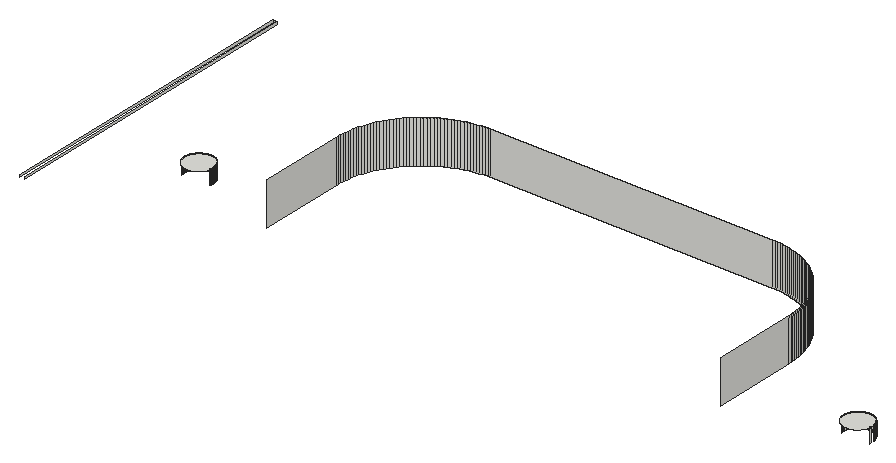
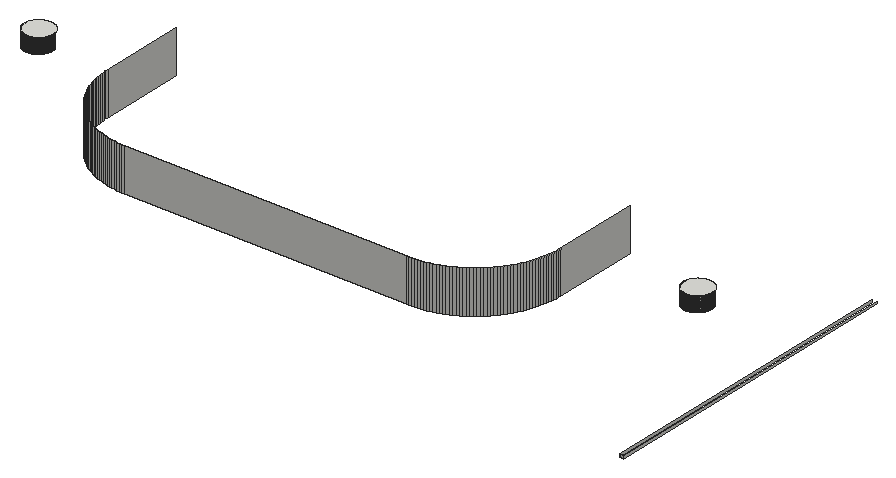
# SketchUp Ruby script. Lengths in inches.
U = 1.inch
M = Sketchup.active_model
def pt(a) = Geom::Point3d.new(a.map { |v| v * U })
def face(e, loops, mat)
  f = e.add_face(loops[0].map { |a| pt(a) })
  loops[1..].each { |l| e.add_face(l.map { |a| pt(a) }).erase! }
  f.material = f.back_material = mat if mat
  f
end
# faces: each face lists its corners as indices into pts; further lists are holes
def faces(e, pts, list, mat = nil) = list.each { |f| face(e, (f[0].is_a?(Array) ? f : [f]).map { |l| l.map { |i| pts[i] } }, mat) }
# xy, xz, yz: faces in a plane at the given z, y or x. An outline is a flat list of corners, or four numbers for a rectangle; further outlines are holes
def ring(l) = l.size == 4 ? [[l[0], l[1]], [l[2], l[1]], [l[2], l[3]], [l[0], l[3]]] : l.each_slice(2).to_a
def flat(e, list, mat, &to3) = list.each { |f| face(e, (f[0].is_a?(Array) ? f : [f]).map { |l| ring(l).map { |u, v| to3.(u, v) } }, mat) }
def xy(e, z, list, mat = nil) = flat(e, list, mat) { |x, y| [x, y, z] }
def xz(e, y, list, mat = nil) = flat(e, list, mat) { |x, z| [x, y, z] }
def yz(e, x, list, mat = nil) = flat(e, list, mat) { |y, z| [x, y, z] }
def lines(e, pts, list) = list.each { |a, b| e.add_line(pt(pts[a]), pt(pts[b])) }
# prism: a flat outline (further loops are holes) pulled along v
def prism(e, loops, v, mat = nil)
  f = face(e, loops, mat); d = Geom::Vector3d.new(v.map { |x| x * U })
  f.pushpull(f.normal.samedirection?(d) ? d.length : -d.length)
end
def box(e, o, s, mat = nil) = prism(e, [[o, [o[0] + s[0], o[1], o[2]], [o[0] + s[0], o[1] + s[1], o[2]], [o[0], o[1] + s[1], o[2]]]], [0, 0, s[2]], mat)
def at(x, y, z, deg = 0) = Geom::Transformation.translation(pt([x, y, z])) * Geom::Transformation.rotation(ORIGIN, Z_AXIS, deg.degrees)
def axes(o, x, y, z) = Geom::Transformation.new([*x, 0, *y, 0, *z, 0, *pt(o).to_a, 1])
def part(name) = M.definitions.add(name)
# library, detail: a bought-in or finely detailed component or shape, given as its bounding box
def library(name, o, s) = part(name).tap { |d| box(d.entities, o, s) }
def detail(e, o, s) = box(e.add_group.entities, o, s)
def put(e, d, t, mat = nil) = e.add_instance(d, t).tap { |i| i.material = mat if mat }
def group(e, t, mat = nil) = e.add_group.tap { |g| g.transformation = t; g.material = mat if mat }.entities
root = M.entities
xy(root,351,[[44.84,249,44.76,249.01,44.6875,249.02,44.61,249.03,44.45,249.05,44.375,249.07,44.3,249.08,44.22,249.1,44.15,249.125,44.07,249.15,44,249.17,43.92,249.2,43.71,249.29,43.64,249.33,43.57,249.36,43.43,249.44,43.37,249.48,43.3,249.53,43.24,249.57,43.17,249.62,42.93,249.82,42.88,249.88,42.77,249.99,42.62,250.17,42.57,250.24,42.53,250.3,42.48,250.37,42.44,250.43,42.36,250.57,42.33,250.64,42.29,250.71,42.23,250.85,42.2,250.93,42.17,251,42.15,251.07,42.125,251.15,42.1,251.22,42.08,251.3,42.07,251.375,42.05,251.45,42.03,251.61,42.02,251.6875,42.01,251.76,42,251.84,42,252.16,42.01,252.24,42.02,252.3125,42.03,252.39,42.05,252.55,42.07,252.625,42.08,252.7,42.1,252.78,42.125,252.85,42.15,252.93,42.17,253,42.2,253.08,42.29,253.29,42.33,253.36,42.36,253.43,42.44,253.57,42.48,253.63,42.53,253.7,42.57,253.76,42.62,253.83,42.82,254.07,42.88,254.12,42.99,254.23,43.17,254.38,43.24,254.43,43.3,254.47,43.37,254.52,43.43,254.56,43.57,254.64,43.64,254.67,43.71,254.71,43.85,254.77,43.93,254.8,44,254.83,44.07,254.85,44.15,254.875,44.22,254.9,44.3,254.92,44.375,254.93,44.45,254.95,44.61,254.97,44.6875,254.98,44.76,254.99,44.84,255,45.16,255,45.24,254.99,45.3125,254.98,45.39,254.97,45.55,254.95,45.625,254.93,45.7,254.92,45.78,254.9,45.85,254.875,45.93,254.85,46,254.83,46.08,254.8,46.29,254.71,46.36,254.67,46.43,254.64,46.57,254.56,46.63,254.52,46.7,254.47,46.76,254.43,46.83,254.38,47.07,254.18,47.12,254.12,47.23,254.01,47.38,253.83,47.43,253.76,47.47,253.7,47.52,253.63,47.56,253.57,47.64,253.43,47.67,253.36,47.71,253.29,47.77,253.15,47.8,253.07,47.83,253,47.85,252.93,47.875,252.85,47.9,252.78,47.92,252.7,47.93,252.625,47.95,252.55,47.97,252.39,47.98,252.3125,47.99,252.24,48,252.16,48,251.84,47.99,251.76,47.98,251.6875,47.97,251.61,47.95,251.45,47.93,251.375,47.92,251.3,47.9,251.22,47.875,251.15,47.85,251.07,47.83,251,47.8,250.92,47.71,250.71,47.67,250.64,47.64,250.57,47.56,250.43,47.52,250.37,47.47,250.3,47.43,250.24,47.38,250.17,47.18,249.93,47.12,249.88,47.01,249.77,46.83,249.62,46.76,249.57,46.7,249.53,46.63,249.48,46.57,249.44,46.43,249.36,46.36,249.33,46.29,249.29,46.15,249.23,46.07,249.2,46,249.17,45.93,249.15,45.85,249.125,45.78,249.1,45.7,249.08,45.625,249.07,45.55,249.05,45.39,249.03,45.3125,249.02,45.24,249.01,45.16,249],[182.84,249,182.76,249.01,182.6875,249.02,182.61,249.03,182.45,249.05,182.375,249.07,182.3,249.08,182.22,249.1,182.15,249.125,182.07,249.15,182,249.17,181.92,249.2,181.71,249.29,181.64,249.33,181.57,249.36,181.43,249.44,181.37,249.48,181.3,249.53,181.24,249.57,181.17,249.62,180.93,249.82,180.88,249.88,180.77,249.99,180.62,250.17,180.57,250.24,180.53,250.3,180.48,250.37,180.44,250.43,180.36,250.57,180.33,250.64,180.29,250.71,180.23,250.85,180.2,250.93,180.17,251,180.15,251.07,180.125,251.15,180.1,251.22,180.08,251.3,180.07,251.375,180.05,251.45,180.03,251.61,180.02,251.6875,180.01,251.76,180,251.84,180,252.16,180.01,252.24,180.02,252.3125,180.03,252.39,180.05,252.55,180.07,252.625,180.08,252.7,180.1,252.78,180.125,252.85,180.15,252.93,180.17,253,180.2,253.08,180.29,253.29,180.33,253.36,180.36,253.43,180.44,253.57,180.48,253.63,180.53,253.7,180.57,253.76,180.62,253.83,180.82,254.07,180.88,254.12,180.99,254.23,181.17,254.38,181.24,254.43,181.3,254.47,181.37,254.52,181.43,254.56,181.57,254.64,181.64,254.67,181.71,254.71,181.85,254.77,181.93,254.8,182,254.83,182.07,254.85,182.15,254.875,182.22,254.9,182.3,254.92,182.375,254.93,182.45,254.95,182.61,254.97,182.6875,254.98,182.76,254.99,182.84,255,183.16,255,183.24,254.99,183.3125,254.98,183.39,254.97,183.55,254.95,183.625,254.93,183.7,254.92,183.78,254.9,183.85,254.875,183.93,254.85,184,254.83,184.08,254.8,184.29,254.71,184.36,254.67,184.43,254.64,184.57,254.56,184.63,254.52,184.7,254.47,184.76,254.43,184.83,254.38,185.07,254.18,185.12,254.12,185.23,254.01,185.38,253.83,185.43,253.76,185.47,253.7,185.52,253.63,185.56,253.57,185.64,253.43,185.67,253.36,185.71,253.29,185.77,253.15,185.8,253.07,185.83,253,185.85,252.93,185.875,252.85,185.9,252.78,185.92,252.7,185.93,252.625,185.95,252.55,185.97,252.39,185.98,252.3125,185.99,252.24,186,252.16,186,251.84,185.99,251.76,185.98,251.6875,185.97,251.61,185.95,251.45,185.93,251.375,185.92,251.3,185.9,251.22,185.875,251.15,185.85,251.07,185.83,251,185.8,250.92,185.71,250.71,185.67,250.64,185.64,250.57,185.56,250.43,185.52,250.37,185.47,250.3,185.43,250.24,185.38,250.17,185.18,249.93,185.12,249.88,185.01,249.77,184.83,249.62,184.76,249.57,184.7,249.53,184.63,249.48,184.57,249.44,184.43,249.36,184.36,249.33,184.29,249.29,184.15,249.23,184.07,249.2,184,249.17,183.93,249.15,183.85,249.125,183.78,249.1,183.7,249.08,183.625,249.07,183.55,249.05,183.39,249.03,183.3125,249.02,183.24,249.01,183.16,249]])
xz(root,255,[[44.84,348,44.92,351],[44.92,348,45,351],[45,348,45.08,351],[45.08,348,45.16,351],[182.84,348,182.92,351],
  [182.92,348,183,351],[183,348,183.08,351],[183.08,348,183.16,351]])
xz(root,282,[[82,348,141,357]])
xz(root,300,[[22,348,23,348.5]])
yz(root,22,[[234,348,300,348.5]])
yz(root,23,[[234,348,300,348.5]])
yz(root,42,[[251.84,348,251.92,351],[251.92,348,252,351],[252,348,252.08,351],[252.08,348,252.16,351]])
yz(root,48,[[251.84,348,251.92,351],[251.92,348,252,351],[252,348,252.08,351],[252.08,348,252.16,351]])
yz(root,64,[[246,348,264,357]])
yz(root,159,[[246,348,264,357]])
yz(root,180,[[251.84,348,251.92,351],[251.92,348,252,351],[252,348,252.08,351],[252.08,348,252.16,351]])
p = [[42.08,251.3,348],[42.07,251.375,348],[42.07,251.375,351],[42.08,251.3,351],[47.93,251.375,348],[47.92,251.3,348],
  [47.92,251.3,351],[47.93,251.375,351],[180.08,251.3,348],[180.07,251.375,348],[180.07,251.375,351],[180.08,251.3,351],
  [42.05,251.45,348],[42.05,251.45,351],[47.95,251.45,348],[47.95,251.45,351],[180.05,251.45,348],[180.05,251.45,351],
  [185.95,251.45,348],[185.93,251.375,348],[185.93,251.375,351],[185.95,251.45,351],[42.04,251.53,348],[42.03,251.61,348],
  [42.03,251.61,351],[42.04,251.53,351],[47.96,251.53,348],[47.96,251.53,351],[47.97,251.61,348],[47.97,251.61,351],
  [180.04,251.53,348],[180.03,251.61,348],[180.03,251.61,351],[180.04,251.53,351],[185.96,251.53,348],[185.96,251.53,351],
  [185.97,251.61,348],[185.97,251.61,351],[42.02,251.6875,348],[42.02,251.6875,351],[47.98,251.6875,348],[47.98,251.6875,351],
  [180.02,251.6875,348],[180.02,251.6875,351],[185.98,251.6875,348],[185.98,251.6875,351],[42.01,251.76,348],[42.01,251.76,351],
  [47.99,251.76,348],[47.99,251.76,351],[180.01,251.76,348],[180.01,251.76,351],[42,251.84,348],[42,251.84,351],
  [48,251.84,348],[48,251.84,351],[180,251.84,348],[180,251.84,351],[42,252.16,348],[42.01,252.24,348],
  [42.01,252.24,351],[42,252.16,351],[42.02,252.3125,348],[42.02,252.3125,351],[47.98,252.3125,348],[47.99,252.24,348],
  [47.99,252.24,351],[47.98,252.3125,351],[48,252.16,348],[48,252.16,351],[180,252.16,348],[180.01,252.24,348],
  [180.01,252.24,351],[180,252.16,351],[180.02,252.3125,348],[180.02,252.3125,351],[42.03,252.39,348],[42.03,252.39,351],
  [47.97,252.39,348],[47.97,252.39,351],[180.03,252.39,348],[180.03,252.39,351],[42.04,252.47,348],[42.04,252.47,351],
  [47.96,252.47,348],[47.96,252.47,351],[180.04,252.47,348],[180.04,252.47,351],[185.96,252.47,348],[185.97,252.39,348],
  [185.97,252.39,351],[185.96,252.47,351],[42.05,252.55,348],[42.05,252.55,351],[42.07,252.625,348],[42.07,252.625,351],
  [47.93,252.625,348],[47.95,252.55,348],[47.95,252.55,351],[47.93,252.625,351],[180.05,252.55,348],[180.05,252.55,351],
  [180.07,252.625,348],[180.07,252.625,351],[185.93,252.625,348],[185.95,252.55,348],[185.95,252.55,351],[185.93,252.625,351],
  [42.08,252.7,348],[42.08,252.7,351],[47.92,252.7,348],[47.92,252.7,351],[180.08,252.7,348],[180.08,252.7,351],
  [185.92,252.7,348],[185.92,252.7,351],[42.1,252.78,348],[42.1,252.78,351],[47.9,252.78,348],[47.9,252.78,351],
  [180.1,252.78,348],[180.1,252.78,351],[185.9,252.78,348],[185.9,252.78,351],[42.125,252.85,348],[42.125,252.85,351],
  [47.875,252.85,348],[47.875,252.85,351],[180.125,252.85,348],[180.125,252.85,351],[185.875,252.85,348],[185.875,252.85,351],
  [42.15,252.93,348],[42.15,252.93,351],[42.17,253,348],[42.17,253,351],[47.83,253,348],[47.85,252.93,348],
  [47.85,252.93,351],[47.83,253,351],[180.15,252.93,348],[180.15,252.93,351],[180.17,253,348],[180.17,253,351],
  [185.83,253,348],[185.85,252.93,348],[185.85,252.93,351],[185.83,253,351],[42.2,253.08,348],[42.2,253.08,351],
  [47.8,253.07,348],[47.8,253.07,351],[180.2,253.08,348],[180.2,253.08,351],[185.8,253.07,348],[185.8,253.07,351],
  [42.23,253.15,348],[42.23,253.15,351],[42.26,253.22,348],[42.26,253.22,351],[47.74,253.22,348],[47.77,253.15,348],
  [47.77,253.15,351],[47.74,253.22,351],[180.23,253.15,348],[180.23,253.15,351],[180.26,253.22,348],[180.26,253.22,351],
  [185.74,253.22,348],[185.77,253.15,348],[185.77,253.15,351],[185.74,253.22,351],[42.29,253.29,348],[42.29,253.29,351],
  [47.71,253.29,348],[47.71,253.29,351],[180.29,253.29,348],[180.29,253.29,351],[185.71,253.29,348],[185.71,253.29,351],
  [42.33,253.36,348],[42.33,253.36,351],[47.67,253.36,348],[47.67,253.36,351],[180.33,253.36,348],[180.33,253.36,351],
  [185.67,253.36,348],[185.67,253.36,351],[42.36,253.43,348],[42.36,253.43,351],[42.4,253.5,348],[42.4,253.5,351],
  [47.6,253.5,348],[47.64,253.43,348],[47.64,253.43,351],[47.6,253.5,351],[180.36,253.43,348],[180.36,253.43,351],
  [180.4,253.5,348],[180.4,253.5,351],[185.6,253.5,348],[185.64,253.43,348],[185.64,253.43,351],[185.6,253.5,351],
  [42.44,253.57,348],[42.44,253.57,351],[47.56,253.57,348],[47.56,253.57,351],[180.44,253.57,348],[180.44,253.57,351],
  [185.56,253.57,348],[185.56,253.57,351],[42.48,253.63,348],[42.48,253.63,351],[42.53,253.7,348],[42.53,253.7,351],
  [47.47,253.7,348],[47.52,253.63,348],[47.52,253.63,351],[47.47,253.7,351],[180.48,253.63,348],[180.48,253.63,351],
  [180.53,253.7,348],[180.53,253.7,351],[185.47,253.7,348],[185.52,253.63,348],[185.52,253.63,351],[185.47,253.7,351],
  [42.57,253.76,348],[42.57,253.76,351],[47.43,253.76,348],[47.43,253.76,351],[180.57,253.76,348],[180.57,253.76,351],
  [185.43,253.76,348],[185.43,253.76,351],[42.62,253.83,348],[42.62,253.83,351],[42.67,253.89,348],[42.67,253.89,351],
  [47.33,253.89,348],[47.38,253.83,348],[47.38,253.83,351],[47.33,253.89,351],[180.62,253.83,348],[180.62,253.83,351],
  [180.67,253.89,348],[180.67,253.89,351],[185.33,253.89,348],[185.38,253.83,348],[185.38,253.83,351],[185.33,253.89,351],
  [42.72,253.95,348],[42.72,253.95,351],[42.77,254.01,348],[42.77,254.01,351],[47.23,254.01,348],[47.28,253.95,348],
  [47.28,253.95,351],[47.23,254.01,351],[180.72,253.95,348],[180.72,253.95,351],[180.77,254.01,348],[180.77,254.01,351],
  [185.23,254.01,348],[185.28,253.95,348],[185.28,253.95,351],[185.23,254.01,351],[42.82,254.07,348],[42.82,254.07,351],
  [47.18,254.06,348],[47.18,254.06,351],[180.82,254.07,348],[180.82,254.07,351],[185.18,254.06,348],[185.18,254.06,351],
  [42.88,254.12,348],[42.88,254.12,351],[42.94,254.18,348],[42.94,254.18,351],[47.07,254.18,348],[47.12,254.12,348],
  [47.12,254.12,351],[47.07,254.18,351],[180.88,254.12,348],[180.88,254.12,351],[180.94,254.18,348],[180.94,254.18,351],
  [185.07,254.18,348],[185.12,254.12,348],[185.12,254.12,351],[185.07,254.18,351],[42.99,254.23,348],[42.99,254.23,351],
  [43.05,254.28,348],[43.05,254.28,351],[46.95,254.28,348],[47.01,254.23,348],[47.01,254.23,351],[46.95,254.28,351],
  [180.99,254.23,348],[180.99,254.23,351],[181.05,254.28,348],[181.05,254.28,351],[184.95,254.28,348],[185.01,254.23,348],
  [185.01,254.23,351],[184.95,254.28,351],[43.11,254.33,348],[43.11,254.33,351],[43.17,254.38,348],[43.17,254.38,351],
  [46.83,254.38,348],[46.89,254.33,348],[46.89,254.33,351],[46.83,254.38,351],[181.11,254.33,348],[181.11,254.33,351],
  [181.17,254.38,348],[181.17,254.38,351],[184.83,254.38,348],[184.89,254.33,348],[184.89,254.33,351],[184.83,254.38,351],
  [43.24,254.43,348],[43.24,254.43,351],[43.3,254.47,348],[43.3,254.47,351],[46.7,254.47,348],[46.76,254.43,348],
  [46.76,254.43,351],[46.7,254.47,351],[181.24,254.43,348],[181.24,254.43,351],[181.3,254.47,348],[181.3,254.47,351],
  [184.7,254.47,348],[184.76,254.43,348],[184.76,254.43,351],[184.7,254.47,351],[43.37,254.52,348],[43.37,254.52,351],
  [43.43,254.56,348],[43.43,254.56,351],[46.57,254.56,348],[46.63,254.52,348],[46.63,254.52,351],[46.57,254.56,351],
  [181.37,254.52,348],[181.37,254.52,351],[181.43,254.56,348],[181.43,254.56,351],[184.57,254.56,348],[184.63,254.52,348],
  [184.63,254.52,351],[184.57,254.56,351],[43.5,254.6,348],[43.5,254.6,351],[43.57,254.64,348],[43.57,254.64,351],
  [43.64,254.67,348],[43.64,254.67,351],[46.36,254.67,348],[46.43,254.64,348],[46.43,254.64,351],[46.36,254.67,351],
  [46.5,254.6,348],[46.5,254.6,351],[181.5,254.6,348],[181.5,254.6,351],[181.57,254.64,348],[181.57,254.64,351],
  [181.64,254.67,348],[181.64,254.67,351],[184.36,254.67,348],[184.43,254.64,348],[184.43,254.64,351],[184.36,254.67,351],
  [184.5,254.6,348],[184.5,254.6,351],[43.71,254.71,348],[43.71,254.71,351],[43.78,254.74,348],[43.78,254.74,351],
  [43.85,254.77,348],[43.85,254.77,351],[46.15,254.77,348],[46.22,254.74,348],[46.22,254.74,351],[46.15,254.77,351],
  [46.29,254.71,348],[46.29,254.71,351],[181.71,254.71,348],[181.71,254.71,351],[181.78,254.74,348],[181.78,254.74,351],
  [181.85,254.77,348],[181.85,254.77,351],[184.15,254.77,348],[184.22,254.74,348],[184.22,254.74,351],[184.15,254.77,351],
  [184.29,254.71,348],[184.29,254.71,351],[43.93,254.8,348],[43.93,254.8,351],[44,254.83,348],[44,254.83,351],
  [44.07,254.85,348],[44.07,254.85,351],[45.93,254.85,348],[46,254.83,348],[46,254.83,351],[45.93,254.85,351],
  [46.08,254.8,348],[46.08,254.8,351],[181.93,254.8,348],[181.93,254.8,351],[182,254.83,348],[182,254.83,351],
  [182.07,254.85,348],[182.07,254.85,351],[183.93,254.85,348],[184,254.83,348],[184,254.83,351],[183.93,254.85,351],
  [184.08,254.8,348],[184.08,254.8,351],[44.15,254.875,348],[44.15,254.875,351],[44.22,254.9,348],[44.22,254.9,351],
  [44.3,254.92,348],[44.3,254.92,351],[44.375,254.93,348],[44.375,254.93,351],[44.45,254.95,348],[44.45,254.95,351],
  [44.53,254.96,348],[44.53,254.96,351],[45.47,254.96,348],[45.55,254.95,348],[45.55,254.95,351],[45.47,254.96,351],
  [45.625,254.93,348],[45.625,254.93,351],[45.7,254.92,348],[45.7,254.92,351],[45.78,254.9,348],[45.78,254.9,351],
  [45.85,254.875,348],[45.85,254.875,351],[182.15,254.875,348],[182.15,254.875,351],[182.22,254.9,348],[182.22,254.9,351],
  [182.3,254.92,348],[182.3,254.92,351],[182.375,254.93,348],[182.375,254.93,351],[182.45,254.95,348],[182.45,254.95,351],
  [182.53,254.96,348],[182.53,254.96,351],[183.47,254.96,348],[183.55,254.95,348],[183.55,254.95,351],[183.47,254.96,351],
  [183.625,254.93,348],[183.625,254.93,351],[183.7,254.92,348],[183.7,254.92,351],[183.78,254.9,348],[183.78,254.9,351],
  [183.85,254.875,348],[183.85,254.875,351],[44.61,254.97,348],[44.61,254.97,351],[44.6875,254.98,348],[44.6875,254.98,351],
  [44.76,254.99,348],[44.76,254.99,351],[44.84,255,348],[44.84,255,351],[45.16,255,348],[45.24,254.99,348],
  [45.24,254.99,351],[45.16,255,351],[45.3125,254.98,348],[45.3125,254.98,351],[45.39,254.97,348],[45.39,254.97,351],
  [182.61,254.97,348],[182.61,254.97,351],[182.6875,254.98,348],[182.6875,254.98,351],[182.76,254.99,348],[182.76,254.99,351],
  [182.84,255,348],[182.84,255,351],[183.16,255,348],[183.24,254.99,348],[183.24,254.99,351],[183.16,255,351],
  [183.3125,254.98,348],[183.3125,254.98,351],[183.39,254.97,348],[183.39,254.97,351],[64.01,264.57,357],[64,264,357],
  [64,264,348],[64.01,264.57,348],[159,264,357],[158.99,264.57,357],[158.99,264.57,348],[159,264,348],
  [64.04,265.13,357],[64.04,265.13,348],[158.96,265.13,357],[158.96,265.13,348],[64.08,265.69,357],[64.08,265.69,348],
  [158.92,265.69,357],[158.92,265.69,348],[64.14,266.26,357],[64.14,266.26,348],[158.86,266.26,357],[158.86,266.26,348],
  [64.22,266.82,357],[64.22,266.82,348],[158.78,266.82,357],[158.78,266.82,348],[64.32,267.37,357],[64.32,267.37,348],
  [158.68,267.37,357],[158.68,267.37,348],[64.43,267.93,357],[64.43,267.93,348],[158.57,267.93,357],[158.57,267.93,348],
  [64.57,268.48,357],[64.57,268.48,348],[158.43,268.48,357],[158.43,268.48,348],[64.71,269.02,357],[64.71,269.02,348],
  [158.29,269.02,357],[158.29,269.02,348],[64.88,269.5625,357],[64.88,269.5625,348],[158.12,269.5625,357],[158.12,269.5625,348],
  [65.0625,270.1,357],[65.0625,270.1,348],[157.9375,270.1,357],[157.9375,270.1,348],[65.26,270.625,357],[65.26,270.625,348],
  [157.74,270.625,357],[157.74,270.625,348],[65.48,271.15,357],[65.48,271.15,348],[157.52,271.15,357],[157.52,271.15,348],
  [65.71,271.66,357],[65.71,271.66,348],[157.29,271.66,357],[157.29,271.66,348],[65.96,272.17,357],[65.96,272.17,348],
  [157.04,272.17,357],[157.04,272.17,348],[66.23,272.67,357],[66.23,272.67,348],[156.77,272.67,357],[156.77,272.67,348],
  [66.51,273.16,357],[66.51,273.16,348],[156.49,273.16,357],[156.49,273.16,348],[66.8,273.64,357],[66.8,273.64,348],
  [156.2,273.64,357],[156.2,273.64,348],[67.11,274.12,357],[67.11,274.12,348],[155.89,274.12,357],[155.89,274.12,348],
  [67.4375,274.58,357],[67.4375,274.58,348],[155.5625,274.58,357],[155.5625,274.58,348],[67.78,275.03,357],[67.78,275.03,348],
  [155.22,275.03,357],[155.22,275.03,348],[68.13,275.47,357],[68.13,275.47,348],[154.87,275.47,357],[154.87,275.47,348],
  [68.5,275.9,357],[68.5,275.9,348],[154.5,275.9,357],[154.5,275.9,348],[68.88,276.32,357],[68.88,276.32,348],
  [154.12,276.32,357],[154.12,276.32,348],[69.27,276.73,357],[69.27,276.73,348],[153.73,276.73,357],[153.73,276.73,348],
  [69.68,277.12,357],[69.68,277.12,348],[153.32,277.12,357],[153.32,277.12,348],[70.1,277.5,357],[70.1,277.5,348],
  [152.9,277.5,357],[152.9,277.5,348],[70.53,277.87,357],[70.53,277.87,348],[152.47,277.87,357],[152.47,277.87,348],
  [70.97,278.22,357],[70.97,278.22,348],[152.03,278.22,357],[152.03,278.22,348],[71.42,278.5625,357],[71.42,278.5625,348],
  [151.58,278.5625,357],[151.58,278.5625,348],[71.88,278.89,357],[71.88,278.89,348],[151.12,278.89,357],[151.12,278.89,348],
  [72.36,279.2,357],[72.36,279.2,348],[150.64,279.2,357],[150.64,279.2,348],[72.84,279.49,357],[72.84,279.49,348],
  [150.16,279.49,357],[150.16,279.49,348],[73.33,279.77,357],[73.33,279.77,348],[149.67,279.77,357],[149.67,279.77,348],
  [73.83,280.04,357],[73.83,280.04,348],[149.17,280.04,357],[149.17,280.04,348],[74.34,280.29,357],[74.34,280.29,348],
  [148.66,280.29,357],[148.66,280.29,348],[74.85,280.52,357],[74.85,280.52,348],[148.15,280.52,357],[148.15,280.52,348],
  [75.375,280.74,357],[75.375,280.74,348],[147.625,280.74,357],[147.625,280.74,348],[75.9,280.9375,357],[75.9,280.9375,348],
  [147.1,280.9375,357],[147.1,280.9375,348],[76.4375,281.12,357],[76.4375,281.12,348],[146.5625,281.12,357],[146.5625,281.12,348],
  [76.98,281.29,357],[76.98,281.29,348],[146.02,281.29,357],[146.02,281.29,348],[77.52,281.43,357],[77.52,281.43,348],
  [145.48,281.43,357],[145.48,281.43,348],[78.07,281.57,357],[78.07,281.57,348],[144.93,281.57,357],[144.93,281.57,348],
  [78.63,281.68,357],[78.63,281.68,348],[144.37,281.68,357],[144.37,281.68,348],[79.18,281.78,357],[79.18,281.78,348],
  [143.82,281.78,357],[143.82,281.78,348],[79.74,281.86,357],[79.74,281.86,348],[143.26,281.86,357],[143.26,281.86,348],
  [80.31,281.92,357],[80.31,281.92,348],[80.87,281.96,357],[80.87,281.96,348],[142.69,281.92,357],[142.13,281.96,357],
  [142.13,281.96,348],[142.69,281.92,348],[81.43,281.99,357],[81.43,281.99,348],[82,282,357],[82,282,348],
  [141.57,281.99,357],[141,282,357],[141,282,348],[141.57,281.99,348]]
faces(root,p,[[0,1,2,3],[4,5,6,7],[8,9,10,11],[1,12,13,2],[14,4,7,15],[9,16,17,10],[18,19,20,21],[22,23,24,25],
  [12,22,25,13],[26,14,15,27],[28,26,27,29],[30,31,32,33],[16,30,33,17],[34,18,21,35],[36,34,35,37],[23,38,39,24],
  [40,28,29,41],[31,42,43,32],[44,36,37,45],[38,46,47,39],[48,40,41,49],[42,50,51,43],[46,52,53,47],[54,48,49,55],
  [50,56,57,51],[58,59,60,61],[59,62,63,60],[64,65,66,67],[65,68,69,66],[70,71,72,73],[71,74,75,72],[62,76,77,63],
  [78,64,67,79],[74,80,81,75],[76,82,83,77],[84,78,79,85],[80,86,87,81],[88,89,90,91],[82,92,93,83],[92,94,95,93],
  [96,97,98,99],[97,84,85,98],[86,100,101,87],[100,102,103,101],[104,105,106,107],[105,88,91,106],[94,108,109,95],[110,96,99,111],
  [102,112,113,103],[114,104,107,115],[108,116,117,109],[118,110,111,119],[112,120,121,113],[122,114,115,123],[116,124,125,117],[126,118,119,127],
  [120,128,129,121],[130,122,123,131],[124,132,133,125],[132,134,135,133],[136,137,138,139],[137,126,127,138],[128,140,141,129],[140,142,143,141],
  [144,145,146,147],[145,130,131,146],[134,148,149,135],[150,136,139,151],[142,152,153,143],[154,144,147,155],[148,156,157,149],[156,158,159,157],
  [160,161,162,163],[161,150,151,162],[152,164,165,153],[164,166,167,165],[168,169,170,171],[169,154,155,170],[158,172,173,159],[174,160,163,175],
  [166,176,177,167],[178,168,171,179],[172,180,181,173],[182,174,175,183],[176,184,185,177],[186,178,179,187],[180,188,189,181],[188,190,191,189],
  [192,193,194,195],[193,182,183,194],[184,196,197,185],[196,198,199,197],[200,201,202,203],[201,186,187,202],[190,204,205,191],[206,192,195,207],
  [198,208,209,199],[210,200,203,211],[204,212,213,205],[212,214,215,213],[216,217,218,219],[217,206,207,218],[208,220,221,209],[220,222,223,221],
  [224,225,226,227],[225,210,211,226],[214,228,229,215],[230,216,219,231],[222,232,233,223],[234,224,227,235],[228,236,237,229],[236,238,239,237],
  [240,241,242,243],[241,230,231,242],[232,244,245,233],[244,246,247,245],[248,249,250,251],[249,234,235,250],[238,252,253,239],[252,254,255,253],
  [256,257,258,259],[257,240,243,258],[246,260,261,247],[260,262,263,261],[264,265,266,267],[265,248,251,266],[254,268,269,255],[270,256,259,271],
  [262,272,273,263],[274,264,267,275],[268,276,277,269],[276,278,279,277],[280,281,282,283],[281,270,271,282],[272,284,285,273],[284,286,287,285],
  [288,289,290,291],[289,274,275,290],[278,292,293,279],[292,294,295,293],[296,297,298,299],[297,280,283,298],[286,300,301,287],[300,302,303,301],
  [304,305,306,307],[305,288,291,306],[294,308,309,295],[308,310,311,309],[312,313,314,315],[313,296,299,314],[302,316,317,303],[316,318,319,317],
  [320,321,322,323],[321,304,307,322],[310,324,325,311],[324,326,327,325],[328,329,330,331],[329,312,315,330],[318,332,333,319],[332,334,335,333],
  [336,337,338,339],[337,320,323,338],[326,340,341,327],[340,342,343,341],[344,345,346,347],[345,328,331,346],[334,348,349,335],[348,350,351,349],
  [352,353,354,355],[353,336,339,354],[342,356,357,343],[356,358,359,357],[358,360,361,359],[362,363,364,365],[363,366,367,364],[366,344,347,367],
  [350,368,369,351],[368,370,371,369],[370,372,373,371],[374,375,376,377],[375,378,379,376],[378,352,355,379],[360,380,381,361],[380,382,383,381],
  [382,384,385,383],[386,387,388,389],[387,390,391,388],[390,362,365,391],[372,392,393,373],[392,394,395,393],[394,396,397,395],[398,399,400,401],
  [399,402,403,400],[402,374,377,403],[384,404,405,385],[404,406,407,405],[406,408,409,407],[410,411,412,413],[411,414,415,412],[414,386,389,415],
  [396,416,417,397],[416,418,419,417],[418,420,421,419],[422,423,424,425],[423,426,427,424],[426,398,401,427],[408,428,429,409],[428,430,431,429],
  [430,432,433,431],[432,434,435,433],[434,436,437,435],[436,438,439,437],[440,441,442,443],[441,444,445,442],[444,446,447,445],[446,448,449,447],
  [448,450,451,449],[450,410,413,451],[420,452,453,421],[452,454,455,453],[454,456,457,455],[456,458,459,457],[458,460,461,459],[460,462,463,461],
  [464,465,466,467],[465,468,469,466],[468,470,471,469],[470,472,473,471],[472,474,475,473],[474,422,425,475],[438,476,477,439],[476,478,479,477],
  [478,480,481,479],[480,482,483,481],[484,485,486,487],[485,488,489,486],[488,490,491,489],[490,440,443,491],[462,492,493,463],[492,494,495,493],
  [494,496,497,495],[496,498,499,497],[500,501,502,503],[501,504,505,502],[504,506,507,505],[506,464,467,507],[508,509,510,511],[512,513,514,515],
  [516,508,511,517],[513,518,519,514],[520,516,517,521],[518,522,523,519],[524,520,521,525],[522,526,527,523],[528,524,525,529],[526,530,531,527],
  [532,528,529,533],[530,534,535,531],[536,532,533,537],[534,538,539,535],[540,536,537,541],[538,542,543,539],[544,540,541,545],[542,546,547,543],
  [548,544,545,549],[546,550,551,547],[552,548,549,553],[550,554,555,551],[556,552,553,557],[554,558,559,555],[560,556,557,561],[558,562,563,559],
  [564,560,561,565],[562,566,567,563],[568,564,565,569],[566,570,571,567],[572,568,569,573],[570,574,575,571],[576,572,573,577],[574,578,579,575],
  [580,576,577,581],[578,582,583,579],[584,580,581,585],[582,586,587,583],[588,584,585,589],[586,590,591,587],[592,588,589,593],[590,594,595,591],
  [596,592,593,597],[594,598,599,595],[600,596,597,601],[598,602,603,599],[604,600,601,605],[602,606,607,603],[608,604,605,609],[606,610,611,607],
  [612,608,609,613],[610,614,615,611],[616,612,613,617],[614,618,619,615],[620,616,617,621],[618,622,623,619],[624,620,621,625],[622,626,627,623],
  [628,624,625,629],[626,630,631,627],[632,628,629,633],[630,634,635,631],[636,632,633,637],[634,638,639,635],[640,636,637,641],[638,642,643,639],
  [644,640,641,645],[642,646,647,643],[648,644,645,649],[646,650,651,647],[652,648,649,653],[650,654,655,651],[656,652,653,657],[654,658,659,655],
  [660,656,657,661],[658,662,663,659],[664,660,661,665],[662,666,667,663],[668,664,665,669],[666,670,671,667],[672,668,669,673],[670,674,675,671],
  [676,672,673,677],[674,678,679,675],[680,676,677,681],[678,682,683,679],[684,680,681,685],[682,686,687,683],[688,684,685,689],[686,690,691,687],
  [692,688,689,693],[690,694,695,691],[696,692,693,697],[698,696,697,699],[700,701,702,703],[694,700,703,695],[704,698,699,705],[706,704,705,707],
  [708,709,710,711],[701,708,711,702]])
